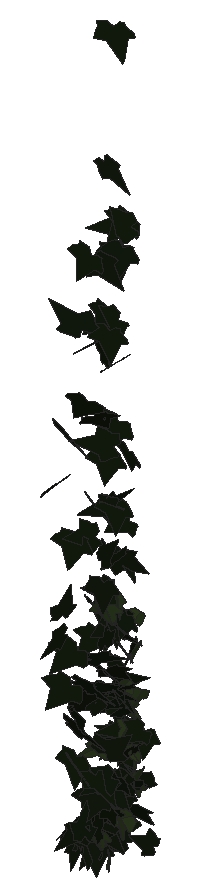
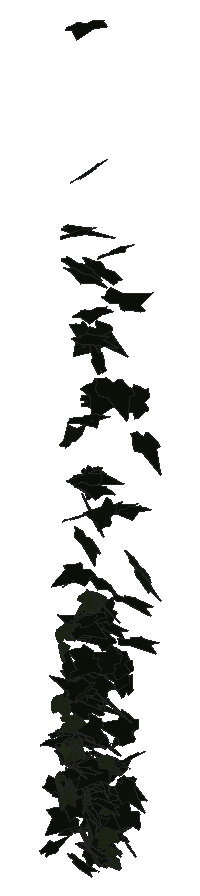
# SketchUp Ruby script. Lengths in inches.
U = 1.inch
M = Sketchup.active_model
def pt(a) = Geom::Point3d.new(a.map { |v| v * U })
def face(e, loops, mat)
  f = e.add_face(loops[0].map { |a| pt(a) })
  loops[1..].each { |l| e.add_face(l.map { |a| pt(a) }).erase! }
  f.material = f.back_material = mat if mat
  f
end
# faces: each face lists its corners as indices into pts; further lists are holes
def faces(e, pts, list, mat = nil) = list.each { |f| face(e, (f[0].is_a?(Array) ? f : [f]).map { |l| l.map { |i| pts[i] } }, mat) }
# xy, xz, yz: faces in a plane at the given z, y or x. An outline is a flat list of corners, or four numbers for a rectangle; further outlines are holes
def ring(l) = l.size == 4 ? [[l[0], l[1]], [l[2], l[1]], [l[2], l[3]], [l[0], l[3]]] : l.each_slice(2).to_a
def flat(e, list, mat, &to3) = list.each { |f| face(e, (f[0].is_a?(Array) ? f : [f]).map { |l| ring(l).map { |u, v| to3.(u, v) } }, mat) }
def xy(e, z, list, mat = nil) = flat(e, list, mat) { |x, y| [x, y, z] }
def xz(e, y, list, mat = nil) = flat(e, list, mat) { |x, z| [x, y, z] }
def yz(e, x, list, mat = nil) = flat(e, list, mat) { |y, z| [x, y, z] }
def lines(e, pts, list) = list.each { |a, b| e.add_line(pt(pts[a]), pt(pts[b])) }
# prism: a flat outline (further loops are holes) pulled along v
def prism(e, loops, v, mat = nil)
  f = face(e, loops, mat); d = Geom::Vector3d.new(v.map { |x| x * U })
  f.pushpull(f.normal.samedirection?(d) ? d.length : -d.length)
end
def box(e, o, s, mat = nil) = prism(e, [[o, [o[0] + s[0], o[1], o[2]], [o[0] + s[0], o[1] + s[1], o[2]], [o[0], o[1] + s[1], o[2]]]], [0, 0, s[2]], mat)
def at(x, y, z, deg = 0) = Geom::Transformation.translation(pt([x, y, z])) * Geom::Transformation.rotation(ORIGIN, Z_AXIS, deg.degrees)
def axes(o, x, y, z) = Geom::Transformation.new([*x, 0, *y, 0, *z, 0, *pt(o).to_a, 1])
def part(name) = M.definitions.add(name)
# library, detail: a bought-in or finely detailed component or shape, given as its bounding box
def library(name, o, s) = part(name).tap { |d| box(d.entities, o, s) }
def detail(e, o, s) = box(e.add_group.entities, o, s)
def put(e, d, t, mat = nil) = e.add_instance(d, t).tap { |i| i.material = mat if mat }
def group(e, t, mat = nil) = e.add_group.tap { |g| g.transformation = t; g.material = mat if mat }.entities
root = M.entities
M.materials.add("1026 AP 7946 SUNNY SIDE UP").color = [254, 231, 186]
M.materials.add("efeu1").color = [18, 25, 13]
M.materials.add("efeu2").color = [43, 57, 29]
c1 = part("ivyleaf_10")
p = [[0,0.5,-0.03],[-0.0625,2.02,-0.43],[-0.19,2.01,-0.46],[-0.54,1.05,-0.29],[-0.52,0.625,-0.18],[-0.83,0.76,-0.28],
  [-1.16,0.64,-0.33],[-1.15,0.33,-0.24],[-0.77,-0.39,0.02],[-0.3,-0.51,0.16],[0.04,-0.48,0.23],[-0.02,2.01,-0.4375],
  [-0.06,2.01,-0.43],[0.04,-0.49,0.23],[0.67,-0.49,0.14],[1.38,0.36,-0.2],[1.375,0.51,-0.24],[0.81,0.65,-0.19],
  [0.62,0.59,-0.15],[0.6,1.09,-0.28],[0.5,1.23,-0.31]]
faces(c1.entities,p,[[0,1,2,3,4,5,6,7,8,9,10],[11,12,0,13,14,15,16,17,18,19,20]],"efeu2")
c2 = part("ivyleaf_9")
p = [[1.54,2.16,1.25],[1.36,2.04,1.19],[-0.21,0.99,0.68],[-0.71,1.11,0.82],[-0.85,0.86,0.67],[-0.8,0.17,0.21],
  [-0.9,-0.01,0.1],[-0.67,-0.16,-0.02],[-0.08,-0.08,-0.05],[-0.03,-0.6,-0.4],[0.65,-0.88,-0.66],[0.83,-0.6,-0.49],
  [1.29,-0.42,-0.43],[1.8125,-0.07,-0.26],[1.21,0.44,0.15]]
faces(c2.entities,p,[[0,1,2,3,4,5,6,7,8,9,10,11,12,13,14]],"efeu1")
put(root,c1,axes([140.67,211.12,291.35],[-0.31101,-0.22054,0.2726],[-0.22025,-0.22884,-0.30425],[0.49649,-0.23967,0.03579]),"1026 AP 7946 SUNNY SIDE UP")
put(root,c1,axes([140.72,211.24,295.79],[0.2323,0.18499,-0.33438],[-0.45552,-0.16539,-0.23317],[-0.3732,0.31702,0.07646]),"1026 AP 7946 SUNNY SIDE UP")
put(root,c1,axes([140.41,211.16,292.48],[-0.21179,-0.31354,-0.22013],[0.17826,0.18116,-0.34932],[0.56771,-0.17385,0.02757]),"1026 AP 7946 SUNNY SIDE UP")
put(root,c2,axes([140.32,210.11,295.625],[-0.15621,-0.45309,0.08274],[0.02346,-0.08791,-0.47717],[0.72389,-0.09492,0.03332]),"1026 AP 7946 SUNNY SIDE UP")
put(root,c2,axes([140.83,208.17,310.09],[-0.19156,0.44772,-0.10637],[0.02533,-0.10522,-0.47847],[-0.72294,-0.12232,0.01142]),"1026 AP 7946 SUNNY SIDE UP")
put(root,c2,axes([140.47,212.01,316.64],[-0.20286,-0.34867,0.24057],[-0.03608,-0.24012,-0.3806],[0.6606,-0.12019,0.05309]),"1026 AP 7946 SUNNY SIDE UP")
put(root,c2,axes([141.02,209.5,317.17],[0.09396,0.14043,0.47018],[-0.74117,0.08625,0.03681],[-0.11241,-0.45133,0.15033]),"1026 AP 7946 SUNNY SIDE UP")
put(root,c2,axes([140,210.16,297.12],[0.51211,-0.2102,0.27942],[0.32542,-0.18001,-0.39903],[0.43225,0.38456,-0.03064]),"1026 AP 7946 SUNNY SIDE UP")
put(root,c2,axes([140.52,212.08,309.62],[-0.44619,-0.27026,-0.14834],[0.20825,0.06639,-0.40113],[0.43289,-0.3105,0.04008]),"1026 AP 7946 SUNNY SIDE UP")
put(root,c2,axes([140.52,209.86,291.53],[-0.3553,-0.02601,-0.29952],[0.44628,-0.10474,-0.21831],[-0.10627,-0.35289,0.08461]),"1026 AP 7946 SUNNY SIDE UP")
put(root,c2,axes([141.11,211.17,303.67],[-0.40313,0.27289,0.15354],[-0.18769,0.08982,-0.38443],[-0.45019,-0.28181,0.02279]),"1026 AP 7946 SUNNY SIDE UP")
put(root,c2,axes([140.54,211.55,297.6],[0.20259,0.08898,0.3734],[0.30588,0.31061,-0.14818],[-0.49992,0.22611,0.06065]),"1026 AP 7946 SUNNY SIDE UP")
put(root,c2,axes([140.51,211.68,295.83],[0.57517,0.18667,0.00256],[0.02196,-0.02424,-0.42223],[-0.2927,0.36499,-0.02665]),"1026 AP 7946 SUNNY SIDE UP")
put(root,c2,axes([141.04,211.95,316.53],[-0.58469,-0.18727,0.19378],[-0.23146,-0.12609,-0.42743],[0.34872,-0.39768,0.0412]),"1026 AP 7946 SUNNY SIDE UP")
put(root,c2,axes([140.73,210.55,320.19],[-0.30714,-0.38459,0.19382],[-0.05448,-0.19429,-0.44224],[0.67252,-0.19138,0.05269]),"1026 AP 7946 SUNNY SIDE UP")
put(root,c2,axes([140.5625,211.22,291.99],[0.15054,0.36754,0.13758],[-0.08456,-0.12165,0.39],[0.60792,-0.10793,0.02018]),"1026 AP 7946 SUNNY SIDE UP")
put(root,c2,axes([140.3,208.92,312.37],[0.58492,-0.27051,0.11828],[0.11594,-0.09591,-0.47316],[0.44827,0.37777,-0.03195]),"1026 AP 7946 SUNNY SIDE UP")
put(root,c2,axes([141.04,209.95,313.38],[0.38137,0.15607,-0.37975],[-0.48213,-0.20625,-0.29829],[-0.40663,0.39092,-0.00248]),"1026 AP 7946 SUNNY SIDE UP")
put(root,c2,axes([140.53,210.78,303.07],[0.54744,-0.18894,-0.07237],[-0.11443,0.01063,-0.4072],[0.29495,0.3548,-0.02367]),"1026 AP 7946 SUNNY SIDE UP")
put(root,c2,axes([140.77,209.24,292.58],[0.30124,0.3797,0.20747],[0.14161,0.17772,-0.43709],[-0.6592,0.21169,0.00092]),"1026 AP 7946 SUNNY SIDE UP")
put(root,c2,axes([140.67,210.85,291.47],[0.05557,0.32279,-0.22727],[0.03544,0.2213,0.33582],[0.61539,-0.0419,0.00118]),"1026 AP 7946 SUNNY SIDE UP")
put(root,c2,axes([141.37,210.51,298.62],[-0.5791,0.28224,0.04961],[-0.11353,-0.01828,-0.47435],[-0.43523,-0.37077,0.05772]),"1026 AP 7946 SUNNY SIDE UP")
put(root,c2,axes([140.4375,211.08,307.75],[0.42116,-0.32124,0.21249],[0.17225,-0.17902,-0.43101],[0.57665,0.28809,-0.02645]),"1026 AP 7946 SUNNY SIDE UP")
put(root,c2,axes([141.1,212.16,295.79],[-0.52423,-0.15829,0.03355],[-0.01562,-0.05649,-0.3775],[0.25392,-0.33027,0.04605]),"1026 AP 7946 SUNNY SIDE UP")
put(root,c2,axes([140.98,211.5625,291.72],[-0.50353,-0.11369,-0.13983],[0.22144,0.00427,-0.34761],[0.16745,-0.34753,0.03923]),"1026 AP 7946 SUNNY SIDE UP")
put(root,c2,axes([141.15,210.88,293.68],[-0.56165,-0.09388,0.0033],[0.00765,-0.03314,-0.37912],[0.14753,-0.35567,0.03221]),"1026 AP 7946 SUNNY SIDE UP")
put(root,c2,axes([140.71,212.21,299.67],[0.21926,-0.36772,0.01179],[-0.01285,-0.01756,-0.405],[0.57846,0.139,-0.01347]),"1026 AP 7946 SUNNY SIDE UP")
put(root,c2,axes([141.15,208.14,303.85],[-0.4997,0.30258,-0.13412],[-0.13728,0.09953,0.45248],[0.50053,0.32937,-0.0098]),"1026 AP 7946 SUNNY SIDE UP")
put(root,c2,axes([141.33,210.66,316.27],[-0.36471,0.30209,-0.26196],[0.02258,-0.29007,-0.36773],[-0.62222,-0.1876,0.1402]),"1026 AP 7946 SUNNY SIDE UP")
put(root,c2,axes([140.7,211.35,315.04],[-0.04949,0.10232,0.46816],[0.16165,-0.44212,0.10744],[0.71347,0.10726,0.00813]),"1026 AP 7946 SUNNY SIDE UP")
put(root,c1,axes([140.89,211.23,303.4375],[-0.25404,0.305,-0.20858],[0.09036,-0.19933,-0.35473],[-0.57002,-0.16752,0.03672]),"1026 AP 7946 SUNNY SIDE UP")
put(root,c2,axes([140.83,211.74,303.07],[-0.04795,-0.39287,-0.14648],[0.01608,0.13958,-0.40513],[0.65557,-0.03216,-0.00078]),"1026 AP 7946 SUNNY SIDE UP")
put(root,c2,axes([141.49,211.96,291.11],[-0.44139,-0.01092,-0.27137],[-0.41313,-0.01921,0.28921],[-0.03319,0.38443,0.009]),"1026 AP 7946 SUNNY SIDE UP")
put(root,c2,axes([140.54,210.64,300.4],[0.34523,-0.24196,0.27913],[0.29074,-0.19994,-0.33776],[0.49354,0.28704,0.00372]),"1026 AP 7946 SUNNY SIDE UP")
put(root,c2,axes([140.9,210.2,291.83],[-0.10088,-0.43975,0.05002],[-0.02052,-0.04968,-0.45807],[0.6958,-0.06522,-0.00626]),"1026 AP 7946 SUNNY SIDE UP")
put(root,c2,axes([140.98,212.19,296.22],[-0.17987,-0.33319,0.15516],[-0.01312,-0.15736,-0.36153],[0.57603,-0.10762,0.04022]),"1026 AP 7946 SUNNY SIDE UP")
put(root,c2,axes([141.5625,211.13,298.47],[-0.57229,0.04186,0.21947],[-0.33997,-0.03741,-0.37359],[-0.02676,-0.41994,0.05266]),"1026 AP 7946 SUNNY SIDE UP")
put(root,c2,axes([140.87,212.18,319.78],[-0.43311,-0.28098,-0.27064],[0.46088,0.05318,-0.37717],[0.38906,-0.3758,0.14551]),"1026 AP 7946 SUNNY SIDE UP")
put(root,c2,axes([140.61,211.15,319.68],[-0.06721,-0.22087,-0.42536],[0.59419,0.22667,-0.16439],[0.43185,-0.34626,0.15999]),"1026 AP 7946 SUNNY SIDE UP")
put(root,c2,axes([141.05,209.14,307.02],[-0.36435,-0.39469,-0.01318],[0.04374,-0.00411,-0.47076],[0.61929,-0.23192,0.02549]),"1026 AP 7946 SUNNY SIDE UP")
put(root,c2,axes([141.23,211.38,291.46],[-0.26291,0.165,-0.2905],[0.21738,-0.25242,-0.2373],[-0.46686,-0.21044,0.0531]),"1026 AP 7946 SUNNY SIDE UP")
put(root,c2,axes([141.22,210.25,291.55],[-0.54687,0.03182,-0.18246],[0.27006,-0.05761,-0.35808],[-0.08537,-0.3861,0.03606]),"1026 AP 7946 SUNNY SIDE UP")
put(root,c2,axes([141.32,208.9375,293.5],[-0.3067,0.29324,-0.27811],[0.1791,-0.24893,-0.36257],[-0.60245,-0.22329,0.0338]),"1026 AP 7946 SUNNY SIDE UP")
put(root,c1,axes([141.27,211.75,292.38],[0.32408,-0.25732,-0.16474],[-0.17601,0.11314,-0.33863],[0.44137,0.23406,-0.01408]),"1026 AP 7946 SUNNY SIDE UP")
put(root,c1,axes([141.12,211.7,294.3125],[0.12909,-0.32823,-0.16526],[0.07012,0.17035,-0.33851],[0.56887,0.05349,0.07922]),"1026 AP 7946 SUNNY SIDE UP")
put(root,c2,axes([141.3,210.3,301.89],[-0.57114,-0.17016,-0.00991],[0.03659,-0.02936,-0.41168],[0.2654,-0.36214,0.03543]),"1026 AP 7946 SUNNY SIDE UP")
put(root,c1,axes([141.18,211.16,292.5],[-0.39451,0.26652,0.02913],[-0.05,0.00678,-0.37657],[-0.41821,-0.25223,0.01754]),"1026 AP 7946 SUNNY SIDE UP")
put(root,c2,axes([141.33,208.39,300.27],[-0.59462,-0.26886,0.061],[-0.0484,-0.06128,-0.47723],[0.4307,-0.37807,0.03059]),"1026 AP 7946 SUNNY SIDE UP")
put(root,c2,axes([141.51,209.82,307.03],[-0.31692,-0.1316,0.38445],[-0.38789,-0.28673,-0.24261],[0.48792,-0.31342,0.05684]),"1026 AP 7946 SUNNY SIDE UP")
put(root,c2,axes([141.45,210.73,299.34],[0.25658,0.30682,-0.23843],[-0.19175,-0.1991,-0.35896],[-0.57482,0.20337,0.01332]),"1026 AP 7946 SUNNY SIDE UP")
put(root,c2,axes([141.51,207.68,303.12],[-0.56976,0.21382,-0.2246],[0.26557,-0.14379,-0.43289],[-0.40169,-0.39835,0.03239]),"1026 AP 7946 SUNNY SIDE UP")
put(root,c2,axes([140.98,211.29,324.49],[0.33134,-0.38477,-0.16321],[-0.01789,0.1698,-0.44557],[0.65275,0.19996,0.07064]),"1026 AP 7946 SUNNY SIDE UP")
put(root,c2,axes([141.28,212.03,320.04],[-0.58004,-0.16132,-0.2536],[0.3887,0.0417,-0.41106],[0.24893,-0.44101,0.05095]),"1026 AP 7946 SUNNY SIDE UP")
put(root,c2,axes([141.54,211.64,302.53],[-0.08842,0.11457,-0.42974],[0.06241,-0.41816,-0.12608],[-0.67833,-0.05341,0.04442]),"1026 AP 7946 SUNNY SIDE UP")
put(root,c2,axes([141.17,208.74,296.34],[0.59233,-0.18047,-0.19198],[-0.27277,0.06663,-0.4297],[0.30174,0.41451,-0.01157]),"1026 AP 7946 SUNNY SIDE UP")
put(root,c2,axes([141.85,211.78,321.46],[-0.61358,-0.01402,0.28139],[-0.40138,-0.15258,-0.38453],[0.15477,-0.45127,0.11832]),"1026 AP 7946 SUNNY SIDE UP")
put(root,c2,axes([141.1,211.05,294.48],[0.27233,-0.30684,-0.19173],[-0.04574,0.19207,-0.35634],[0.56101,0.16461,0.06402]),"1026 AP 7946 SUNNY SIDE UP")
put(root,c1,axes([141.77,211.67,296.67],[-0.32577,0.10446,0.31166],[-0.46822,0.06727,-0.23408],[-0.18205,-0.35994,0.04434]),"1026 AP 7946 SUNNY SIDE UP")
put(root,c2,axes([141.26,212.18,295.68],[-0.12665,-0.34119,-0.16037],[0.06752,0.14779,-0.36021],[0.58454,-0.09099,0.00686]),"1026 AP 7946 SUNNY SIDE UP")
put(root,c2,axes([141.14,209.0625,298.25],[-0.06249,-0.03067,0.44778],[0.19092,-0.42013,-0.02155],[0.6583,0.11893,0.04876]),"1026 AP 7946 SUNNY SIDE UP")
put(root,c2,axes([141.53,212.12,293.92],[-0.15623,0.13703,-0.34638],[0.20643,-0.31231,-0.17252],[-0.5335,-0.16097,0.03468]),"1026 AP 7946 SUNNY SIDE UP")
put(root,c2,axes([141.18,212.24,305.02],[0.10851,-0.39997,-0.01099],[0.03297,0.01213,-0.41741],[0.62819,0.06845,0.02381]),"1026 AP 7946 SUNNY SIDE UP")
put(root,c2,axes([141.15,209.04,299.01],[0.21846,0.07836,0.45802],[0.52842,0.29197,-0.15966],[-0.47297,0.36239,0.03319]),"1026 AP 7946 SUNNY SIDE UP")
put(root,c2,axes([140.93,209.53,299.77],[0.58267,-0.08396,0.22107],[0.31026,-0.096,-0.38941],[0.18849,0.41756,-0.0424]),"1026 AP 7946 SUNNY SIDE UP")
put(root,c2,axes([141.05,210.3,292.11],[0.0088,-0.03124,0.40222],[0.4129,-0.28966,-0.02944],[0.45734,0.26211,0.01884]),"1026 AP 7946 SUNNY SIDE UP")
put(root,c2,axes([141.68,208.33,302.15],[-0.69139,-0.15138,-0.018],[0.04818,-0.03822,-0.47694],[0.23456,-0.43836,0.04491]),"1026 AP 7946 SUNNY SIDE UP")
put(root,c2,axes([141.54,212.13,321.49],[-0.39653,-0.32475,0.21217],[-0.10379,-0.20826,-0.41906],[0.59727,-0.25179,0.06804]),"1026 AP 7946 SUNNY SIDE UP")
put(root,c2,axes([141.35,210.09,291.76],[-0.40483,-0.2745,-0.21928],[0.26703,0.12944,-0.38565],[0.47475,-0.30688,0.02993]),"1026 AP 7946 SUNNY SIDE UP")
put(root,c2,axes([141.35,210.66,304.26],[-0.46478,-0.15323,-0.3018],[0.48195,0.01727,-0.32879],[0.19158,-0.41519,0.09494]),"1026 AP 7946 SUNNY SIDE UP")
put(root,c2,axes([141.98,210.34,294.74],[-0.10235,0.31789,0.31912],[-0.35368,0.24432,-0.30736],[-0.59938,-0.19846,0.12688]),"1026 AP 7946 SUNNY SIDE UP")
put(root,c2,axes([141.69,208.79,293.24],[-0.03372,0.05467,-0.48628],[0.13688,-0.46438,-0.06216],[-0.73503,-0.08899,0.01073]),"1026 AP 7946 SUNNY SIDE UP")
put(root,c2,axes([141.98,211.76,296.85],[-0.51371,-0.03677,0.23403],[-0.34629,-0.06574,-0.33732],[0.1061,-0.39258,0.03218]),"1026 AP 7946 SUNNY SIDE UP")
put(root,c2,axes([141.52,209.85,312.84],[0.39842,0.37949,0.04753],[0.05841,0.02806,-0.46965],[-0.59785,0.25564,-0.01421]),"1026 AP 7946 SUNNY SIDE UP")
put(root,c1,axes([141.35,211.98,297.85],[-0.46404,-0.05589,-0.25107],[0.3847,0.01082,-0.3081],[0.0787,-0.38238,0.02569]),"1026 AP 7946 SUNNY SIDE UP")
put(root,c2,axes([141.6875,210.875,302.17],[-0.33032,-0.19057,0.30816],[-0.17199,-0.29715,-0.27491],[0.53202,-0.21438,0.10246]),"1026 AP 7946 SUNNY SIDE UP")
put(root,c1,axes([141.5625,210.58,303.2],[-0.55691,-0.17083,-0.09623],[0.15048,0.01382,-0.40396],[0.26578,-0.36578,0.02707]),"1026 AP 7946 SUNNY SIDE UP")
put(root,c1,axes([141.53,211.48,303.26],[-0.08386,0.37267,-0.14765],[0.01862,-0.14519,-0.38859],[-0.62876,-0.054,0.00819]),"1026 AP 7946 SUNNY SIDE UP")
put(root,c2,axes([141.4,211.71,305.08],[0.0532,-0.06411,-0.43225],[0.01251,0.42057,-0.06314],[0.66673,-0.00278,0.03567]),"1026 AP 7946 SUNNY SIDE UP")
put(root,c2,axes([142.17,211.71,296.72],[-0.40736,0.07095,0.31891],[-0.49198,0.00839,-0.27205],[-0.0819,-0.40327,0.04801]),"1026 AP 7946 SUNNY SIDE UP")
put(root,c2,axes([141.93,212.01,292.39],[-0.36623,-0.07397,0.29219],[-0.32637,-0.21489,-0.23424],[0.32634,-0.29792,0.09365]),"1026 AP 7946 SUNNY SIDE UP")
put(root,c2,axes([141.46,211.27,331.27],[-0.15707,-0.43855,-0.17987],[0.08692,0.16381,-0.46209],[0.73566,-0.11299,0.01619]),"1026 AP 7946 SUNNY SIDE UP")
put(root,c2,axes([141.24,211.69,299.16],[0.10726,0.00499,0.39753],[0.5913,-0.08878,-0.06782],[0.13616,0.38165,-0.01862]),"1026 AP 7946 SUNNY SIDE UP")
put(root,c2,axes([141.46,210.95,297.95],[0.59988,0.20671,0.11097],[-0.1907,0.00218,0.44301],[0.31201,-0.3961,0.0574]),"1026 AP 7946 SUNNY SIDE UP")
put(root,c2,axes([141.73,211.15,312.08],[-0.43167,-0.38656,0.04628],[-0.00528,-0.05529,-0.48784],[0.6123,-0.273,0.02841]),"1026 AP 7946 SUNNY SIDE UP")
put(root,c2,axes([141.43,210.35,292.46],[-0.07669,-0.18177,-0.37474],[0.22872,0.33322,-0.19023],[0.59555,-0.15137,0.0248]),"1026 AP 7946 SUNNY SIDE UP")
put(root,c2,axes([141.29,210.51,299.2],[0.55473,0.08782,0.24634],[0.37033,0.04098,-0.37401],[-0.15072,0.42394,-0.01227]),"1026 AP 7946 SUNNY SIDE UP")
put(root,c1,axes([141.74,209.74,292.6],[-0.58065,0.02488,-0.04914],[0.07094,-0.03877,-0.37977],[-0.04644,-0.37034,0.03425]),"1026 AP 7946 SUNNY SIDE UP")
put(root,c2,axes([142.09,212.08,296.14],[-0.37782,0.28261,-0.0167],[-0.07594,-0.06392,-0.37396],[-0.43873,-0.23231,0.07911]),"1026 AP 7946 SUNNY SIDE UP")
put(root,c2,axes([141.63,209.61,293.29],[0.30043,0.31604,0.26407],[0.25883,0.19679,-0.37786],[-0.58322,0.25014,-0.03166]),"1026 AP 7946 SUNNY SIDE UP")
put(root,c1,axes([141.74,212.3,296.23],[-0.14583,-0.00896,-0.40059],[-0.03692,-0.39885,0.0129],[-0.6104,0.02626,0.09492]),"1026 AP 7946 SUNNY SIDE UP")
put(root,c2,axes([142.33,211.17,294.6],[-0.29095,-0.0397,-0.37172],[-0.5247,-0.1402,0.19148],[-0.22381,0.38029,0.03433]),"1026 AP 7946 SUNNY SIDE UP")
put(root,c2,axes([141.93,211.68,294.27],[0.25047,0.31856,-0.15535],[-0.11245,-0.13485,-0.3677],[-0.54391,0.17458,0.00448]),"1026 AP 7946 SUNNY SIDE UP")
put(root,c2,axes([141.74,212.3,300.78],[-0.19744,0.03794,-0.4089],[0.45466,-0.27818,-0.12319],[-0.43218,-0.30999,0.05721]),"1026 AP 7946 SUNNY SIDE UP")
put(root,c1,axes([141.87,211.99,294.93],[0.3936,-0.28695,-0.04118],[-0.05822,0.01854,-0.39184],[0.45147,0.25256,-0.01463]),"1026 AP 7946 SUNNY SIDE UP")
put(root,c1,axes([141.9,211.5625,296.33],[0.46422,-0.24287,-0.07093],[-0.11404,0.01767,-0.39235],[0.37959,0.30233,-0.03113]),"1026 AP 7946 SUNNY SIDE UP")
put(root,c1,axes([141.91,212.26,302.23],[-0.22779,-0.24304,0.28517],[0.00643,-0.29986,-0.26944],[0.58082,-0.092,0.11483]),"1026 AP 7946 SUNNY SIDE UP")
put(root,c1,axes([141.73,211.73,296.87],[-0.09709,-0.11934,0.38343],[0.24233,-0.35442,-0.09264],[0.5659,0.13129,0.10545]),"1026 AP 7946 SUNNY SIDE UP")
put(root,c2,axes([141.88,210.2,293.46],[0.34408,0.3254,-0.10343],[-0.06489,-0.09533,-0.40409],[-0.53238,0.22193,-0.01759]),"1026 AP 7946 SUNNY SIDE UP")
put(root,c2,axes([142.15,210.42,305.78],[-0.06478,0.3909,0.20345],[-0.10794,0.18791,-0.40135],[-0.67854,-0.06721,0.04442]),"1026 AP 7946 SUNNY SIDE UP")
put(root,c2,axes([141.71,211.04,302.39],[-0.05988,-0.39261,0.06813],[0.00548,-0.069,-0.40664],[0.62661,-0.03691,0.01007]),"1026 AP 7946 SUNNY SIDE UP")
put(root,c1,axes([141.94,211.54,299.21],[0.08537,0.2475,-0.31156],[-0.18397,-0.28251,-0.26027],[-0.5881,0.1243,0.03619]),"1026 AP 7946 SUNNY SIDE UP")
put(root,c2,axes([141.59,210.59,296.14],[-0.29888,0.08326,0.38309],[0.57761,-0.06852,0.20911],[0.15663,0.41154,-0.04012]),"1026 AP 7946 SUNNY SIDE UP")
put(root,c1,axes([141.9,212.09,294.27],[-0.54232,0.15334,-0.0282],[0.01934,-0.04159,-0.38761],[-0.24441,-0.34354,0.0319]),"1026 AP 7946 SUNNY SIDE UP")
put(root,c2,axes([141.54,210.85,301.95],[0.56993,-0.27405,-0.02934],[-0.06709,-0.01192,-0.46678],[0.42777,0.36326,-0.03411]),"1026 AP 7946 SUNNY SIDE UP")
put(root,c2,axes([141.73,210.57,300.21],[0.45668,0.28369,0.11515],[0.14467,0.06331,-0.41746],[-0.45614,0.30411,-0.01711]),"1026 AP 7946 SUNNY SIDE UP")
put(root,c2,axes([141.56,209.74,301.06],[0.38756,0.13681,0.34253],[0.43054,0.18838,-0.28853],[-0.36464,0.36783,0.02338]),"1026 AP 7946 SUNNY SIDE UP")
put(root,c2,axes([142.19,210.39,293.36],[-0.20047,0.38151,-0.02543],[-0.00641,-0.02966,-0.41434],[-0.60133,-0.12687,0.01289]),"1026 AP 7946 SUNNY SIDE UP")
put(root,c2,axes([142.11,209.82,301.98],[0.13812,0.10836,0.41876],[-0.08592,0.41407,-0.09928],[-0.65494,-0.03147,0.10134]),"1026 AP 7946 SUNNY SIDE UP")
put(root,c2,axes([142.04,211.45,307.26],[-0.41394,-0.20887,0.25743],[-0.10476,-0.28135,-0.31474],[0.50274,-0.23061,0.14637]),"1026 AP 7946 SUNNY SIDE UP")
put(root,c2,axes([141.77,211.11,299.12],[0.39077,-0.27186,-0.21049],[-0.21371,0.15049,-0.37857],[0.48858,0.28325,0.00276]),"1026 AP 7946 SUNNY SIDE UP")
put(root,c2,axes([141.875,211.58,302.45],[-0.14472,-0.34859,0.17942],[-0.02781,-0.17706,-0.37155],[0.6135,-0.09025,0.02548]),"1026 AP 7946 SUNNY SIDE UP")
put(root,c2,axes([141.86,210.44,316.9],[-0.2295,-0.41846,-0.0931],[0.0616,0.0795,-0.45597],[0.66955,-0.15075,0.01004]),"1026 AP 7946 SUNNY SIDE UP")
put(root,c2,axes([141.49,211.11,302],[0.33609,-0.18412,0.30658],[0.38186,-0.17473,-0.29106],[0.39812,0.32302,0.02036]),"1026 AP 7946 SUNNY SIDE UP")
put(root,c2,axes([142.3125,212.03,294.2],[0.20551,0.03077,0.39029],[-0.58986,0.07387,0.12763],[-0.09461,-0.39373,0.05204]),"1026 AP 7946 SUNNY SIDE UP")
put(root,c2,axes([142.11,211.375,293.96],[-0.02224,-0.13601,-0.39148],[0.15296,-0.36939,0.13058],[-0.61475,-0.08699,0.04665]),"1026 AP 7946 SUNNY SIDE UP")
put(root,c2,axes([141.81,210.28,308.45],[0.16217,0.04821,0.44216],[0.45279,0.32083,-0.1066],[-0.50558,0.30279,0.04636]),"1026 AP 7946 SUNNY SIDE UP")
put(root,c1,axes([142.09,211.58,294.78],[0.00529,-0.39384,0.00098],[0.00741,-0.00315,-0.40573],[0.61925,0.0034,0.00484]),"1026 AP 7946 SUNNY SIDE UP")
put(root,c2,axes([142.36,210.18,308.63],[-0.09061,-0.11275,-0.44604],[-0.10254,-0.42912,0.12174],[-0.69501,0.07801,0.04019]),"1026 AP 7946 SUNNY SIDE UP")
put(root,c2,axes([141.99,210.93,299.2],[0.33574,0.28524,0.22154],[0.12165,0.20577,-0.36183],[-0.5468,0.22092,0.05554]),"1026 AP 7946 SUNNY SIDE UP")
put(root,c2,axes([142.09,209.25,294.78],[-0.59997,-0.17512,-0.15855],[0.27292,-0.01906,-0.42381],[0.24321,-0.41062,0.08445]),"1026 AP 7946 SUNNY SIDE UP")
put(root,c1,axes([141.78,211.72,296.1],[0.44684,0.16647,0.2053],[0.27135,0.09779,-0.33871],[-0.30356,0.33246,-0.00057]),"1026 AP 7946 SUNNY SIDE UP")
put(root,c2,axes([141.84,210.48,294.47],[-0.02024,-0.23619,-0.33175],[0.09273,0.31619,-0.2405],[0.61935,-0.05506,0.02516]),"1026 AP 7946 SUNNY SIDE UP")
put(root,c2,axes([142.3,210.43,295.22],[0.37948,0.00881,-0.33933],[-0.50964,-0.06756,-0.24686],[-0.0938,0.40275,-0.03156]),"1026 AP 7946 SUNNY SIDE UP")
put(root,c2,axes([142.13,210.18,315.42],[0.27297,0.31895,0.31764],[0.10614,0.30633,-0.36596],[-0.68743,0.17395,0.06963]),"1026 AP 7946 SUNNY SIDE UP")
put(root,c2,axes([142.61,209.625,311.9],[-0.41974,-0.02136,0.39695],[-0.56748,-0.1525,-0.26709],[0.21541,-0.44335,0.06985]),"1026 AP 7946 SUNNY SIDE UP")
put(root,c1,axes([142.25,212.08,298.64],[-0.22521,-0.3406,0.13344],[-0.03345,-0.13319,-0.38015],[0.57309,-0.14162,0.03025]),"1026 AP 7946 SUNNY SIDE UP")
put(root,c1,axes([141.93,210.34,291.25],[0.06287,-0.07665,0.37054],[0.35292,-0.28207,-0.08918],[0.45892,0.22741,0.01782]),"1026 AP 7946 SUNNY SIDE UP")
put(root,c2,axes([142.21,209.37,293.08],[-0.0802,-0.01169,0.42982],[-0.26454,-0.38416,-0.03451],[0.60073,-0.17073,0.04218]),"1026 AP 7946 SUNNY SIDE UP")
put(root,c2,axes([142.5,209.39,294.38],[0.30448,-0.0122,-0.42473],[-0.64055,-0.07651,-0.19526],[-0.10089,0.44895,-0.04211]),"1026 AP 7946 SUNNY SIDE UP")
put(root,c2,axes([142.27,208.22,293.39],[-0.27419,-0.23076,0.38304],[0.3544,0.29735,0.29971],[-0.59184,0.28497,0.00202]),"1026 AP 7946 SUNNY SIDE UP")
put(root,c2,axes([142.375,211.47,296.23],[-0.13955,0.27251,-0.24753],[0.09329,-0.23476,-0.29635],[-0.56523,-0.10603,0.0122]),"1026 AP 7946 SUNNY SIDE UP")
put(root,c2,axes([141.98,211.83,292.98],[0.54856,0.13202,0.02909],[0.05768,-0.01954,-0.38304],[-0.20404,0.3494,-0.03007]),"1026 AP 7946 SUNNY SIDE UP")
put(root,c1,axes([142.29,212.04,294.8],[0.08619,-0.37083,0.07006],[-0.00388,-0.0712,-0.38637],[0.59341,0.05339,-0.0127]),"1026 AP 7946 SUNNY SIDE UP")
put(root,c1,axes([142.29,211.85,301.01],[0.14123,-0.37953,0.05461],[-0.00172,-0.05691,-0.40186],[0.60305,0.08872,-0.01394]),"1026 AP 7946 SUNNY SIDE UP")
put(root,c2,axes([142.04,209.77,306.12],[-0.1563,0.3118,0.33598],[0.11729,-0.31616,0.3348],[0.69767,0.12301,0.01899]),"1026 AP 7946 SUNNY SIDE UP")
put(root,c2,axes([142.48,211.9,296.97],[-0.35596,-0.23485,0.19086],[-0.18821,-0.14363,-0.33666],[0.43248,-0.25581,0.01058]),"1026 AP 7946 SUNNY SIDE UP")
put(root,c2,axes([142.71,209.39,295.78],[-0.70553,0.06632,-0.02421],[0.02697,-0.04654,-0.46539],[-0.10751,-0.44691,0.04217]),"1026 AP 7946 SUNNY SIDE UP")
put(root,c1,axes([142.72,210.58,293.375],[0.3906,-0.10099,-0.30255],[-0.44137,0.08618,-0.27516],[0.20694,0.37442,-0.0158]),"1026 AP 7946 SUNNY SIDE UP")
put(root,c2,axes([142.35,210.28,308.72],[-0.20943,-0.42901,-0.03321],[0.03249,0.02477,-0.46246],[0.67543,-0.13422,0.01195]),"1026 AP 7946 SUNNY SIDE UP")
put(root,c1,axes([142.4375,210.41,293.17],[-0.34751,0.26824,-0.1307],[0.06849,-0.12905,-0.35574],[-0.46257,-0.22063,0.04552]),"1026 AP 7946 SUNNY SIDE UP")
put(root,c2,axes([142.15,209.22,295.74],[0.05356,-0.43708,-0.11464],[0.24172,0.11384,-0.42089],[0.66571,-0.00617,0.16205]),"1026 AP 7946 SUNNY SIDE UP")
put(root,c2,axes([142.43,212.17,296.75],[-0.19017,-0.38515,-0.00691],[0.01358,0.00203,-0.4158],[0.6055,-0.12101,0.00715]),"1026 AP 7946 SUNNY SIDE UP")
put(root,c2,axes([142.29,211.2,310.87],[-0.02864,-0.31539,0.31158],[0.12814,-0.30163,-0.31887],[0.67704,0.04374,0.07353]),"1026 AP 7946 SUNNY SIDE UP")
put(root,c2,axes([142.79,212.2,291.24],[-0.1051,0.06422,0.38276],[-0.44625,-0.25646,-0.00844],[0.38947,-0.27652,0.09362]),"1026 AP 7946 SUNNY SIDE UP")
